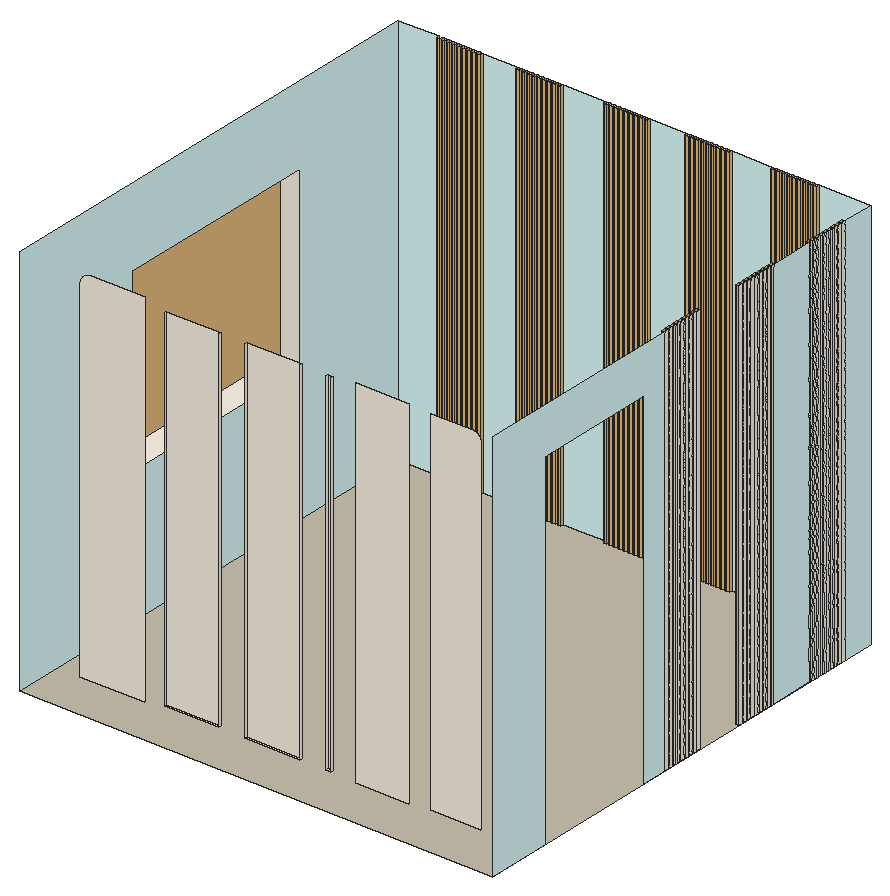
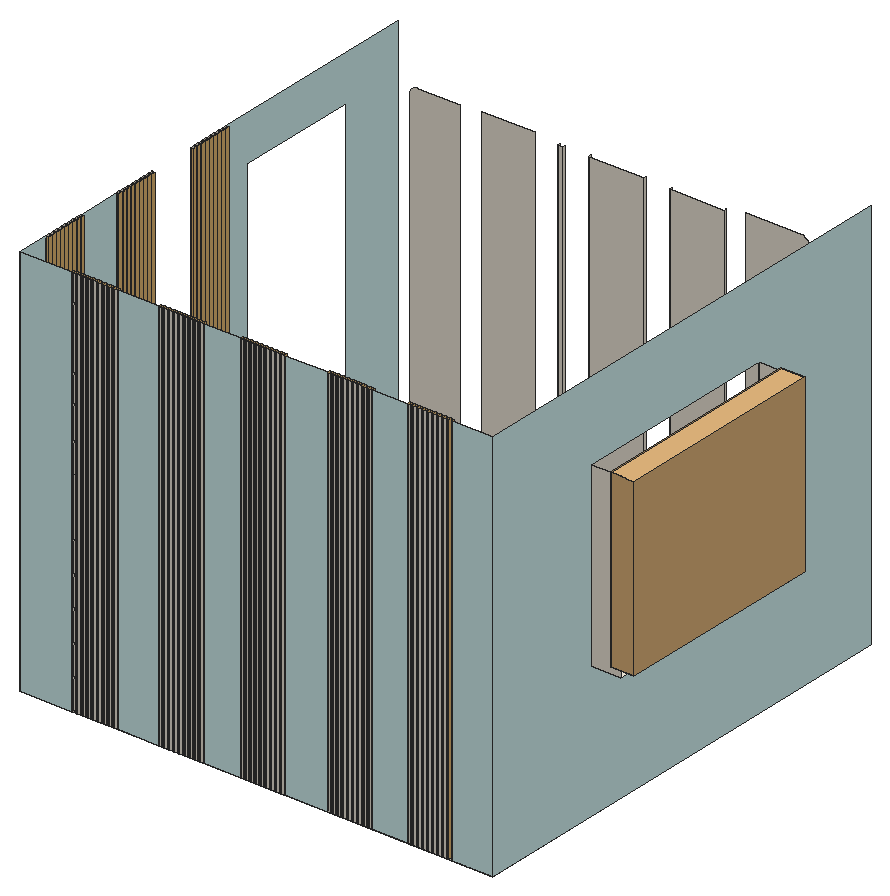
# SketchUp Ruby script. Lengths in inches.
U = 1.inch
M = Sketchup.active_model
def pt(a) = Geom::Point3d.new(a.map { |v| v * U })
def face(e, loops, mat)
  f = e.add_face(loops[0].map { |a| pt(a) })
  loops[1..].each { |l| e.add_face(l.map { |a| pt(a) }).erase! }
  f.material = f.back_material = mat if mat
  f
end
# faces: each face lists its corners as indices into pts; further lists are holes
def faces(e, pts, list, mat = nil) = list.each { |f| face(e, (f[0].is_a?(Array) ? f : [f]).map { |l| l.map { |i| pts[i] } }, mat) }
# xy, xz, yz: faces in a plane at the given z, y or x. An outline is a flat list of corners, or four numbers for a rectangle; further outlines are holes
def ring(l) = l.size == 4 ? [[l[0], l[1]], [l[2], l[1]], [l[2], l[3]], [l[0], l[3]]] : l.each_slice(2).to_a
def flat(e, list, mat, &to3) = list.each { |f| face(e, (f[0].is_a?(Array) ? f : [f]).map { |l| ring(l).map { |u, v| to3.(u, v) } }, mat) }
def xy(e, z, list, mat = nil) = flat(e, list, mat) { |x, y| [x, y, z] }
def xz(e, y, list, mat = nil) = flat(e, list, mat) { |x, z| [x, y, z] }
def yz(e, x, list, mat = nil) = flat(e, list, mat) { |y, z| [x, y, z] }
def lines(e, pts, list) = list.each { |a, b| e.add_line(pt(pts[a]), pt(pts[b])) }
# prism: a flat outline (further loops are holes) pulled along v
def prism(e, loops, v, mat = nil)
  f = face(e, loops, mat); d = Geom::Vector3d.new(v.map { |x| x * U })
  f.pushpull(f.normal.samedirection?(d) ? d.length : -d.length)
end
def box(e, o, s, mat = nil) = prism(e, [[o, [o[0] + s[0], o[1], o[2]], [o[0] + s[0], o[1] + s[1], o[2]], [o[0], o[1] + s[1], o[2]]]], [0, 0, s[2]], mat)
def at(x, y, z, deg = 0) = Geom::Transformation.translation(pt([x, y, z])) * Geom::Transformation.rotation(ORIGIN, Z_AXIS, deg.degrees)
def axes(o, x, y, z) = Geom::Transformation.new([*x, 0, *y, 0, *z, 0, *pt(o).to_a, 1])
def part(name) = M.definitions.add(name)
# library, detail: a bought-in or finely detailed component or shape, given as its bounding box
def library(name, o, s) = part(name).tap { |d| box(d.entities, o, s) }
def detail(e, o, s) = box(e.add_group.entities, o, s)
def put(e, d, t, mat = nil) = e.add_instance(d, t).tap { |i| i.material = mat if mat }
def group(e, t, mat = nil) = e.add_group.tap { |g| g.transformation = t; g.material = mat if mat }.entities
root = M.entities
M.materials.add("[0030_OldLace]").color = [253, 245, 230]
M.materials.add("[0090_LightCyan]").color = [224, 255, 255]
M.materials.add("[Tile Canvas]").color = [199, 192, 173]
M.materials.add("[Wood OSB]").color = [240, 195, 122]
c1 = library("Window 82-25",[-14.97,-2.34,0.01],[29.93,4.71,56.48])
xy(root,3.6,[[68.98,402.03,85.78,402.71]],"[0030_OldLace]")
xy(root,3.73,[[93.66,402.03,95.34,402.71]],"[0030_OldLace]")
xy(root,3.87,[[44.51,402.03,61.02,402.71]],"[0030_OldLace]")
xy(root,41,[[0,434.03,9,497.9]],"[0030_OldLace]")
xz(root,402.71,[[18.24,2.2,18.24,109.45,18.27,109.89,18.36,110.32,18.5,110.74,18.69,111.13,18.9375,111.49,19.22,111.82,19.55,112.11,19.92,112.36,20.3125,112.55,20.73,112.69,21.16,112.78,21.59,112.8,37.94,112.8,37.94,2.2],[102.43,2.87,118.59,112.13],[125.33,3.39,125.33,111.61,137.86,111.61,138.21,111.59,138.56,111.52,138.89,111.41,139.21,111.25,139.5,111.06,139.76,110.83,140,110.5625,140.19,110.27,140.35,109.95,140.46,109.62,140.53,109.28,140.55,108.93,140.55,3.39],[68.98,3.6,85.78,111.4],[93.66,3.73,95.34,111.27],
  [44.51,3.87,61.02,111.13]],"[0030_OldLace]")
xz(root,434.03,[[0,41,9,96]],"[0030_OldLace]")
xz(root,457.1,[[152.125,0,153,120]],"[Wood OSB]")
xz(root,458.18,[[152.125,0,153,120]],"[Wood OSB]")
xz(root,458.65,[[152.125,0,153,120]],"[Wood OSB]")
xz(root,459.73,[[152.125,0,153,120]],"[Wood OSB]")
xz(root,460.19,[[152.125,0,153,120]],"[Wood OSB]")
xz(root,461.27,[[152.125,0,153,120]],"[Wood OSB]")
xz(root,461.74,[[152.125,0,153,120]],"[Wood OSB]")
xz(root,462.82,[[152.125,0,153,120]],"[Wood OSB]")
xz(root,463.29,[[152.125,0,153,120]],"[Wood OSB]")
xz(root,464.37,[[152.125,0,153,120]],"[Wood OSB]")
xz(root,464.83,[[152.125,0,153,120]],"[Wood OSB]")
xz(root,465.91,[[152.125,0,153,120]],"[Wood OSB]")
xz(root,466.38,[[152.125,0,153,120]],"[Wood OSB]")
xz(root,467.46,[[152.125,0,153,120]],"[Wood OSB]")
xz(root,467.93,[[152.125,0,153,120]],"[Wood OSB]")
xz(root,469.01,[[152.125,0,153,120]],"[Wood OSB]")
xz(root,469.48,[[152.125,0,153,120]],"[Wood OSB]")
xz(root,470.55,[[152.125,0,153,120]],"[Wood OSB]")
xz(root,485.35,[[152.125,0,153,120]],"[Wood OSB]")
xz(root,486.43,[[152.125,0,153,120]],"[Wood OSB]")
xz(root,486.9,[[152.125,0,153,120]],"[Wood OSB]")
xz(root,487.98,[[152.125,0,153,120]],"[Wood OSB]")
xz(root,488.44,[[152.125,0,153,120]],"[Wood OSB]")
xz(root,489.52,[[152.125,0,153,120]],"[Wood OSB]")
xz(root,489.99,[[152.125,0,153,120]],"[Wood OSB]")
xz(root,491.07,[[152.125,0,153,120]],"[Wood OSB]")
xz(root,491.54,[[152.125,0,153,120]],"[Wood OSB]")
xz(root,492.62,[[152.125,0,153,120]],"[Wood OSB]")
xz(root,493.08,[[152.125,0,153,120]],"[Wood OSB]")
xz(root,494.16,[[152.125,0,153,120]],"[Wood OSB]")
xz(root,494.63,[[152.125,0,153,120]],"[Wood OSB]")
xz(root,495.71,[[152.125,0,153,120]],"[Wood OSB]")
xz(root,496.18,[[152.125,0,153,120]],"[Wood OSB]")
xz(root,497.26,[[152.125,0,153,120]],"[Wood OSB]")
xz(root,497.73,[[152.125,0,153,120]],"[Wood OSB]")
xz(root,497.9,[[0,41,9,96]],"[0030_OldLace]")
xz(root,498.8,[[152.125,0,153,120]],"[Wood OSB]")
xz(root,512.16,[[152.125,0,153,120]],"[Wood OSB]")
xz(root,513.24,[[152.125,0,153,120]],"[Wood OSB]")
xz(root,513.71,[[152.125,0,153,120]],"[Wood OSB]")
xz(root,514.79,[[152.125,0,153,120]],"[Wood OSB]")
xz(root,515.26,[[152.125,0,153,120]],"[Wood OSB]")
xz(root,516.34,[[152.125,0,153,120]],"[Wood OSB]")
xz(root,516.8,[[152.125,0,153,120]],"[Wood OSB]")
xz(root,517.88,[[152.125,0,153,120]],"[Wood OSB]")
xz(root,518.35,[[152.125,0,153,120]],"[Wood OSB]")
xz(root,519.43,[[152.125,0,153,120]],"[Wood OSB]")
xz(root,519.9,[[152.125,0,153,120]],"[Wood OSB]")
xz(root,520.98,[[152.125,0,153,120]],"[Wood OSB]")
xz(root,521.44,[[152.125,0,153,120]],"[Wood OSB]")
xz(root,522.52,[[152.125,0,153,120]],"[Wood OSB]")
xz(root,522.99,[[152.125,0,153,120]],"[Wood OSB]")
xz(root,524.07,[[152.125,0,153,120]],"[Wood OSB]")
xz(root,524.54,[[152.125,0,153,120]],"[Wood OSB]")
xz(root,525.62,[[152.125,0,153,120]],"[Wood OSB]")
xz(root,534.59,[[21.4,0,22.48,120],[22.95,0,24.03,120],[24.5,0,25.58,120],[26.05,0,27.125,120],[27.59,0,28.67,120],
  [29.14,0,30.22,120],[30.6875,0,31.77,120],[32.23,0,33.3125,120],[33.78,0,34.86,120],[45.72,0,46.8,120],
  [47.29,0,48.37,120],[48.86,0,49.9375,120],[50.43,0,51.51,120],[52,0,53.08,120],[53.57,0,54.65,120],
  [55.14,0,56.22,120],[56.71,0,57.79,120],[58.28,0,59.36,120],[72.4,0,73.48,120],[73.95,0,75.03,120],
  [75.5,0,76.58,120],[77.05,0,78.125,120],[78.59,0,79.67,120],[80.14,0,81.22,120],[81.6875,0,82.77,120],
  [83.23,0,84.3125,120],[84.78,0,85.86,120],[97.15,0,98.23,120],[98.73,0,99.8,120],[100.3,0,101.375,120],
  [101.87,0,102.95,120],[103.4375,0,104.52,120],[105.01,0,106.09,120],[106.58,0,107.66,120],[108.15,0,109.23,120],
  [109.72,0,110.8,120],[123.34,0,124.42,120],[124.94,0,126.02,120],[126.55,0,127.625,120],[128.15,0,129.23,120],
  [129.75,0,130.83,120],[131.35,0,132.43,120],[132.95,0,134.03,120],[134.55,0,135.63,120],[136.15,0,137.23,120]],"[Wood OSB]")
xz(root,535.46,[[22.48,0,22.95,120],[22.95,0,24.03,120],[24.03,0,24.5,120],[24.5,0,25.58,120],[25.58,0,26.05,120],
  [26.05,0,27.125,120],[27.125,0,27.59,120],[27.59,0,28.67,120],[28.67,0,29.14,120],[29.14,0,30.22,120],
  [30.22,0,30.6875,120],[30.6875,0,31.77,120],[31.77,0,32.23,120],[32.23,0,33.3125,120],[33.3125,0,33.78,120],
  [33.78,0,34.8125,120],[34.8125,0,34.86,120],[45.72,0,46.8,120],[46.8,0,47.29,120],[47.29,0,48.37,120],
  [48.37,0,48.86,120],[48.86,0,49.9375,120],[49.9375,0,50.43,120],[50.43,0,51.51,120],[51.51,0,52,120],
  [52,0,53.08,120],[53.08,0,53.57,120],[53.57,0,54.65,120],[54.65,0,55.14,120],[55.14,0,56.22,120],
  [56.22,0,56.71,120],[56.71,0,57.79,120],[57.79,0,58.28,120],[58.28,0,59.125,120],[59.125,0,59.36,120],
  [72.4,0,73.48,120],[73.48,0,73.95,120],[73.95,0,75.03,120],[75.03,0,75.5,120],[75.5,0,76.58,120],
  [76.58,0,77.05,120],[77.05,0,78.125,120],[78.125,0,78.59,120],[78.59,0,79.67,120],[79.67,0,80.14,120],
  [80.14,0,81.22,120],[81.22,0,81.6875,120],[81.6875,0,82.77,120],[82.77,0,83.23,120],[83.23,0,84.3125,120],
  [84.3125,0,84.78,120],[84.78,0,85.8125,120],[85.8125,0,85.86,120],[97.15,0,98.23,120],[98.23,0,98.73,120],
  [98.73,0,99.8,120],[99.8,0,100.3,120],[100.3,0,101.375,120],[101.375,0,101.87,120],[101.87,0,102.95,120],
  [102.95,0,103.4375,120],[103.4375,0,104.52,120],[104.52,0,105.01,120],[105.01,0,106.09,120],[106.09,0,106.58,120],
  [106.58,0,107.66,120],[107.66,0,108.15,120],[108.15,0,109.23,120],[109.23,0,109.72,120],[109.72,0,110.5625,120],
  [110.5625,0,110.8,120],[123.34,0,124.42,120],[124.42,0,124.94,120],[124.94,0,126.02,120],[126.02,0,126.55,120],
  [126.55,0,127.625,120],[127.625,0,128.15,120],[128.15,0,129.23,120],[129.23,0,129.75,120],[129.75,0,130.83,120],
  [130.83,0,131.35,120],[131.35,0,132.43,120],[132.43,0,132.95,120],[132.95,0,134.03,120],[134.03,0,134.55,120],
  [134.55,0,135.63,120],[135.63,0,136.15,120],[136.15,0,136.75,120],[136.75,0,137.23,120]],"[0030_OldLace]")
xz(root,535.46,[[9,0,21.4,120],[34.86,0,45.72,120],[59.36,0,72.4,120],[85.86,0,97.15,120],[110.8,0,123.34,120],
  [137.23,0,153,120]],"[0090_LightCyan]")
yz(root,9,[[[391.46,0,535.46,120],[434.03,41,497.9,96]]],"[0090_LightCyan]")
yz(root,21.4,[[534.59,0,535.46,120]],"[Wood OSB]")
yz(root,22.48,[[534.59,0,535.46,120]],"[Wood OSB]")
yz(root,22.95,[[534.59,0,535.46,120]],"[Wood OSB]")
yz(root,24.03,[[534.59,0,535.46,120]],"[Wood OSB]")
yz(root,24.5,[[534.59,0,535.46,120]],"[Wood OSB]")
yz(root,25.58,[[534.59,0,535.46,120]],"[Wood OSB]")
yz(root,26.05,[[534.59,0,535.46,120]],"[Wood OSB]")
yz(root,27.125,[[534.59,0,535.46,120]],"[Wood OSB]")
yz(root,27.59,[[534.59,0,535.46,120]],"[Wood OSB]")
yz(root,28.67,[[534.59,0,535.46,120]],"[Wood OSB]")
yz(root,29.14,[[534.59,0,535.46,120]],"[Wood OSB]")
yz(root,30.22,[[534.59,0,535.46,120]],"[Wood OSB]")
yz(root,30.6875,[[534.59,0,535.46,120]],"[Wood OSB]")
yz(root,31.77,[[534.59,0,535.46,120]],"[Wood OSB]")
yz(root,32.23,[[534.59,0,535.46,120]],"[Wood OSB]")
yz(root,33.3125,[[534.59,0,535.46,120]],"[Wood OSB]")
yz(root,33.78,[[534.59,0,535.46,120]],"[Wood OSB]")
yz(root,34.86,[[534.59,0,535.46,120]],"[Wood OSB]")
yz(root,44.51,[[402.03,3.87,402.71,111.13]],"[0030_OldLace]")
yz(root,45.72,[[534.59,0,535.46,120]],"[Wood OSB]")
yz(root,46.8,[[534.59,0,535.46,120]],"[Wood OSB]")
yz(root,47.29,[[534.59,0,535.46,120]],"[Wood OSB]")
yz(root,48.37,[[534.59,0,535.46,120]],"[Wood OSB]")
yz(root,48.86,[[534.59,0,535.46,120]],"[Wood OSB]")
yz(root,49.9375,[[534.59,0,535.46,120]],"[Wood OSB]")
yz(root,50.43,[[534.59,0,535.46,120]],"[Wood OSB]")
yz(root,51.51,[[534.59,0,535.46,120]],"[Wood OSB]")
yz(root,52,[[534.59,0,535.46,120]],"[Wood OSB]")
yz(root,53.08,[[534.59,0,535.46,120]],"[Wood OSB]")
yz(root,53.57,[[534.59,0,535.46,120]],"[Wood OSB]")
yz(root,54.65,[[534.59,0,535.46,120]],"[Wood OSB]")
yz(root,55.14,[[534.59,0,535.46,120]],"[Wood OSB]")
yz(root,56.22,[[534.59,0,535.46,120]],"[Wood OSB]")
yz(root,56.71,[[534.59,0,535.46,120]],"[Wood OSB]")
yz(root,57.79,[[534.59,0,535.46,120]],"[Wood OSB]")
yz(root,58.28,[[534.59,0,535.46,120]],"[Wood OSB]")
yz(root,59.36,[[534.59,0,535.46,120]],"[Wood OSB]")
yz(root,61.02,[[402.03,3.87,402.71,111.13]],"[0030_OldLace]")
yz(root,68.98,[[402.03,3.6,402.71,111.4]],"[0030_OldLace]")
yz(root,72.4,[[534.59,0,535.46,120]],"[Wood OSB]")
yz(root,73.48,[[534.59,0,535.46,120]],"[Wood OSB]")
yz(root,73.95,[[534.59,0,535.46,120]],"[Wood OSB]")
yz(root,75.03,[[534.59,0,535.46,120]],"[Wood OSB]")
yz(root,75.5,[[534.59,0,535.46,120]],"[Wood OSB]")
yz(root,76.58,[[534.59,0,535.46,120]],"[Wood OSB]")
yz(root,77.05,[[534.59,0,535.46,120]],"[Wood OSB]")
yz(root,78.125,[[534.59,0,535.46,120]],"[Wood OSB]")
yz(root,78.59,[[534.59,0,535.46,120]],"[Wood OSB]")
yz(root,79.67,[[534.59,0,535.46,120]],"[Wood OSB]")
yz(root,80.14,[[534.59,0,535.46,120]],"[Wood OSB]")
yz(root,81.22,[[534.59,0,535.46,120]],"[Wood OSB]")
yz(root,81.6875,[[534.59,0,535.46,120]],"[Wood OSB]")
yz(root,82.77,[[534.59,0,535.46,120]],"[Wood OSB]")
yz(root,83.23,[[534.59,0,535.46,120]],"[Wood OSB]")
yz(root,84.3125,[[534.59,0,535.46,120]],"[Wood OSB]")
yz(root,84.78,[[534.59,0,535.46,120]],"[Wood OSB]")
yz(root,85.78,[[402.03,3.6,402.71,111.4]],"[0030_OldLace]")
yz(root,85.86,[[534.59,0,535.46,120]],"[Wood OSB]")
yz(root,93.66,[[402.03,3.73,402.71,111.27]],"[0030_OldLace]")
yz(root,95.34,[[402.03,3.73,402.71,111.27]],"[0030_OldLace]")
yz(root,97.15,[[534.59,0,535.46,120]],"[Wood OSB]")
yz(root,98.23,[[534.59,0,535.46,120]],"[Wood OSB]")
yz(root,98.73,[[534.59,0,535.46,120]],"[Wood OSB]")
yz(root,99.8,[[534.59,0,535.46,120]],"[Wood OSB]")
yz(root,100.3,[[534.59,0,535.46,120]],"[Wood OSB]")
yz(root,101.375,[[534.59,0,535.46,120]],"[Wood OSB]")
yz(root,101.87,[[534.59,0,535.46,120]],"[Wood OSB]")
yz(root,102.95,[[534.59,0,535.46,120]],"[Wood OSB]")
yz(root,103.4375,[[534.59,0,535.46,120]],"[Wood OSB]")
yz(root,104.52,[[534.59,0,535.46,120]],"[Wood OSB]")
yz(root,105.01,[[534.59,0,535.46,120]],"[Wood OSB]")
yz(root,106.09,[[534.59,0,535.46,120]],"[Wood OSB]")
yz(root,106.58,[[534.59,0,535.46,120]],"[Wood OSB]")
yz(root,107.66,[[534.59,0,535.46,120]],"[Wood OSB]")
yz(root,108.15,[[534.59,0,535.46,120]],"[Wood OSB]")
yz(root,109.23,[[534.59,0,535.46,120]],"[Wood OSB]")
yz(root,109.72,[[534.59,0,535.46,120]],"[Wood OSB]")
yz(root,110.8,[[534.59,0,535.46,120]],"[Wood OSB]")
yz(root,123.34,[[534.59,0,535.46,120]],"[Wood OSB]")
yz(root,124.42,[[534.59,0,535.46,120]],"[Wood OSB]")
yz(root,124.94,[[534.59,0,535.46,120]],"[Wood OSB]")
yz(root,126.02,[[534.59,0,535.46,120]],"[Wood OSB]")
yz(root,126.55,[[534.59,0,535.46,120]],"[Wood OSB]")
yz(root,127.625,[[534.59,0,535.46,120]],"[Wood OSB]")
yz(root,128.15,[[534.59,0,535.46,120]],"[Wood OSB]")
yz(root,129.23,[[534.59,0,535.46,120]],"[Wood OSB]")
yz(root,129.75,[[534.59,0,535.46,120]],"[Wood OSB]")
yz(root,130.83,[[534.59,0,535.46,120]],"[Wood OSB]")
yz(root,131.35,[[534.59,0,535.46,120]],"[Wood OSB]")
yz(root,132.43,[[534.59,0,535.46,120]],"[Wood OSB]")
yz(root,132.95,[[534.59,0,535.46,120]],"[Wood OSB]")
yz(root,134.03,[[534.59,0,535.46,120]],"[Wood OSB]")
yz(root,134.55,[[534.59,0,535.46,120]],"[Wood OSB]")
yz(root,135.63,[[534.59,0,535.46,120]],"[Wood OSB]")
yz(root,136.15,[[534.59,0,535.46,120]],"[Wood OSB]")
yz(root,137.23,[[534.59,0,535.46,120]],"[Wood OSB]")
yz(root,152.125,[[457.1,0,458.18,120],[458.65,0,459.73,120],[460.19,0,461.27,120],[461.74,0,462.82,120],[463.29,0,464.37,120],
  [464.83,0,465.91,120],[466.38,0,467.46,120],[467.93,0,469.01,120],[469.48,0,470.55,120],[485.35,0,486.43,120],
  [486.9,0,487.98,120],[488.44,0,489.52,120],[489.99,0,491.07,120],[491.54,0,492.62,120],[493.08,0,494.16,120],
  [494.63,0,495.71,120],[496.18,0,497.26,120],[497.73,0,498.8,120],[512.16,0,513.24,120],[513.71,0,514.79,120],
  [515.26,0,516.34,120],[516.8,0,517.88,120],[518.35,0,519.43,120],[519.9,0,520.98,120],[521.44,0,522.52,120],
  [522.99,0,524.07,120],[524.54,0,525.62,120]],"[Wood OSB]")
yz(root,153,[[457.15,0,458.18,120],[458.18,0,458.65,120],[458.65,0,459.73,120],[459.73,0,460.19,120],[460.19,0,461.27,120],
  [461.27,0,461.74,120],[461.74,0,462.82,120],[462.82,0,463.29,120],[463.29,0,464.37,120],[464.37,0,464.83,120],
  [464.83,0,465.91,120],[465.91,0,466.38,120],[466.38,0,467.46,120],[467.46,0,467.93,120],[467.93,0,469.01,120],
  [469.48,0,470.55,120],[485.4,0,486.43,120],[486.43,0,486.9,120],[486.9,0,487.98,120],[487.98,0,488.44,120],
  [488.44,0,489.52,120],[489.52,0,489.99,120],[489.99,0,491.07,120],[491.07,0,491.54,120],[491.54,0,492.62,120],
  [492.62,0,493.08,120],[493.08,0,494.16,120],[494.16,0,494.63,120],[494.63,0,495.71,120],[495.71,0,496.18,120],
  [496.18,0,497.26,120],[497.73,0,498.8,120],[512.16,0,512.21,120],[512.21,0,513.24,120],[513.24,0,513.71,120],
  [513.71,0,514.79,120],[514.79,0,515.26,120],[515.26,0,516.34,120],[516.34,0,516.8,120],[516.8,0,517.88,120],
  [517.88,0,518.35,120],[518.35,0,519.43,120],[519.43,0,519.9,120],[519.9,0,520.98,120],[520.98,0,521.44,120],
  [521.44,0,522.52,120],[522.52,0,522.99,120],[522.99,0,524.07,120],[524.07,0,524.54,120],[524.54,0,525.62,120]],"[0030_OldLace]")
yz(root,153,[[391.46,0,391.46,120,457.1,120,457.1,0,449.03,0,449.03,106,411.21,106,411.21,0],[498.8,0,512.16,120],[525.62,0,535.46,120]],"[0090_LightCyan]")
put(root,c1,axes([-0.64,465.46,42.94],[0,-2.16701,0],[1.5096,0,0],[0,0,0.93941]))
g1 = group(root,at(9,391.46,0),"[Tile Canvas]")
xy(g1,0,[[0,0,144,144]])
